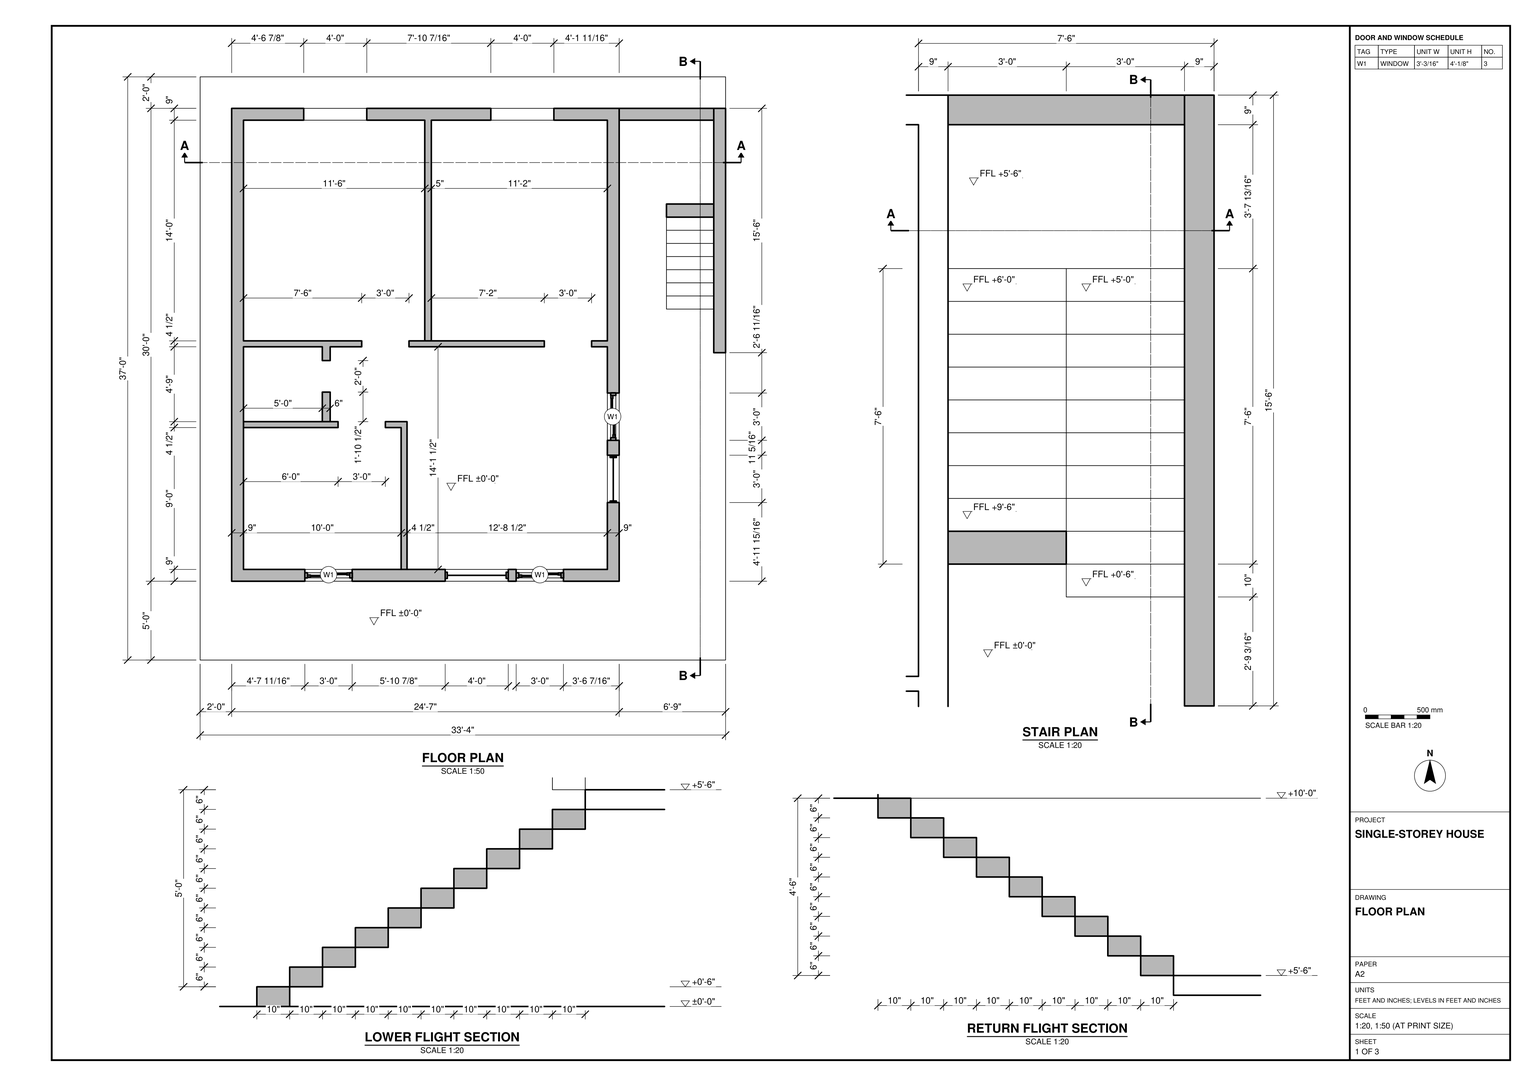
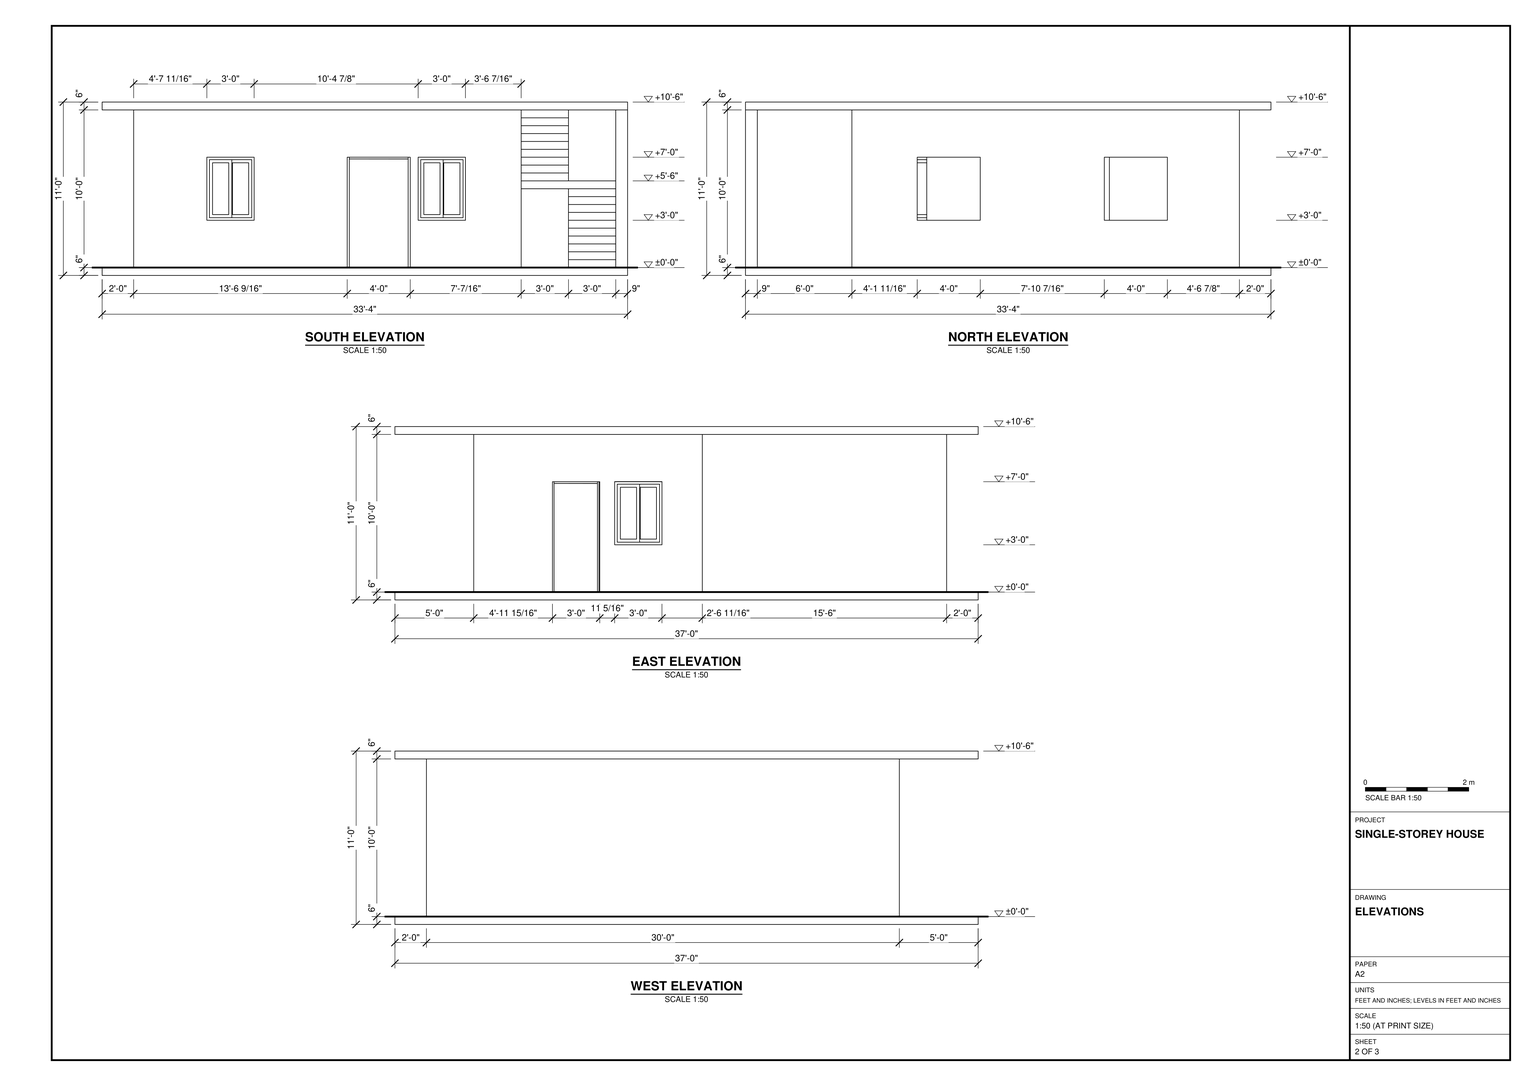
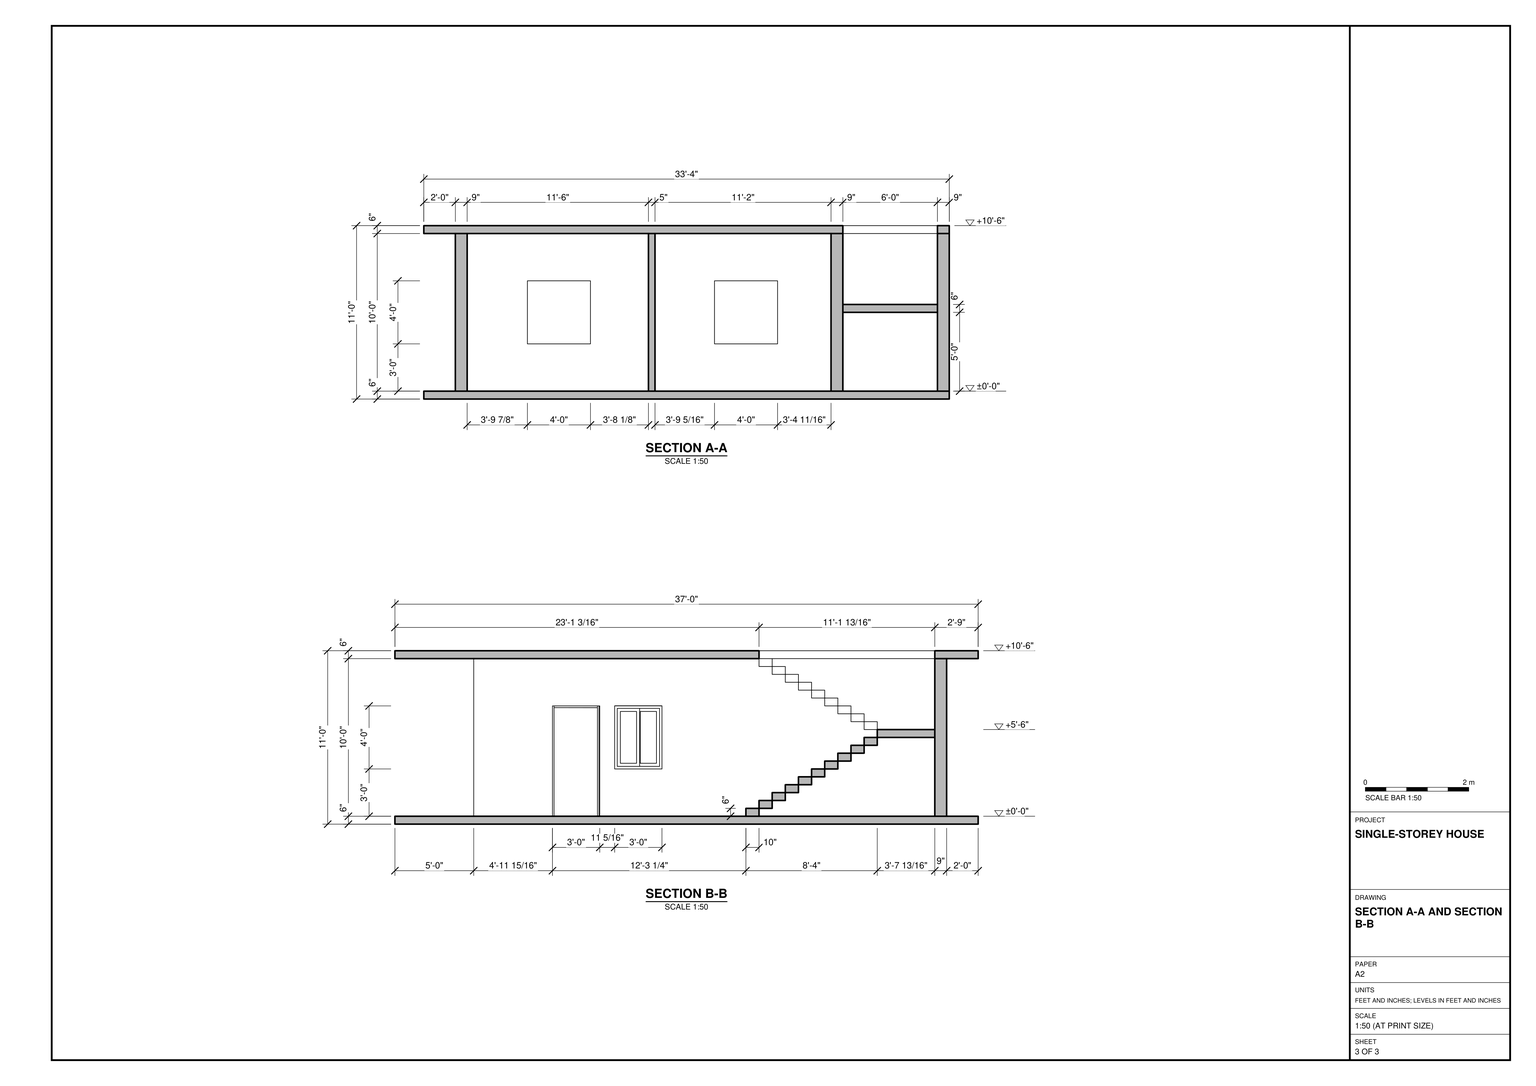
Build the single-storey house in SketchUp from task_files/diagram_01.pdf. Work in feet and inches. The overall dimensions, including the projecting slabs, are 33'-4" east to west, 37'-0" north to south and 11'-0" high. Use ±0'-0" as the finished ground-floor level.

Set out the 24'-7" by 30'-0" enclosed house on the floor slab. Follow the plan for the two rooms across the north end, the smaller subdivided spaces on the west and the larger space at the southeast. Use 9" exterior walls and follow the individual partition thicknesses, including the 5" divider between the north rooms. Cut the passage openings through the partitions. Place the south entrance between two sliding windows, with another doorway and sliding window on the east wall. Reproduce the two plain openings on the north elevation and leave the west wall uninterrupted.

Model the floor slab and flat roof slab, including their projections beyond the walls. At the northeast, build the stair between the house and the outer stair wall. Use the stair plan and sections to connect the parallel flights at the +5'-6" landing and form the roof opening for the return flight.

Keep walls, slabs, roof, stair and any individual furniture or joinery pieces in separate groups or components. Use components for repeated parts. Any decor or loose items may be suitable library components. Save one SketchUp model as output_files/single_storey_house_with_an_external_return_stair.skp.

# SketchUp Ruby script. Lengths in inches.
U = 1.inch
M = Sketchup.active_model
def pt(a) = Geom::Point3d.new(a.map { |v| v * U })
def face(e, loops, mat)
  f = e.add_face(loops[0].map { |a| pt(a) })
  loops[1..].each { |l| e.add_face(l.map { |a| pt(a) }).erase! }
  f.material = f.back_material = mat if mat
  f
end
# faces: each face lists its corners as indices into pts; further lists are holes
def faces(e, pts, list, mat = nil) = list.each { |f| face(e, (f[0].is_a?(Array) ? f : [f]).map { |l| l.map { |i| pts[i] } }, mat) }
# xy, xz, yz: faces in a plane at the given z, y or x. An outline is a flat list of corners, or four numbers for a rectangle; further outlines are holes
def ring(l) = l.size == 4 ? [[l[0], l[1]], [l[2], l[1]], [l[2], l[3]], [l[0], l[3]]] : l.each_slice(2).to_a
def flat(e, list, mat, &to3) = list.each { |f| face(e, (f[0].is_a?(Array) ? f : [f]).map { |l| ring(l).map { |u, v| to3.(u, v) } }, mat) }
def xy(e, z, list, mat = nil) = flat(e, list, mat) { |x, y| [x, y, z] }
def xz(e, y, list, mat = nil) = flat(e, list, mat) { |x, z| [x, y, z] }
def yz(e, x, list, mat = nil) = flat(e, list, mat) { |y, z| [x, y, z] }
def lines(e, pts, list) = list.each { |a, b| e.add_line(pt(pts[a]), pt(pts[b])) }
# prism: a flat outline (further loops are holes) pulled along v
def prism(e, loops, v, mat = nil)
  f = face(e, loops, mat); d = Geom::Vector3d.new(v.map { |x| x * U })
  f.pushpull(f.normal.samedirection?(d) ? d.length : -d.length)
end
def box(e, o, s, mat = nil) = prism(e, [[o, [o[0] + s[0], o[1], o[2]], [o[0] + s[0], o[1] + s[1], o[2]], [o[0], o[1] + s[1], o[2]]]], [0, 0, s[2]], mat)
def at(x, y, z, deg = 0) = Geom::Transformation.translation(pt([x, y, z])) * Geom::Transformation.rotation(ORIGIN, Z_AXIS, deg.degrees)
def axes(o, x, y, z) = Geom::Transformation.new([*x, 0, *y, 0, *z, 0, *pt(o).to_a, 1])
def part(name) = M.definitions.add(name)
# library, detail: a bought-in or finely detailed component or shape, given as its bounding box
def library(name, o, s) = part(name).tap { |d| box(d.entities, o, s) }
def detail(e, o, s) = box(e.add_group.entities, o, s)
def put(e, d, t, mat = nil) = e.add_instance(d, t).tap { |i| i.material = mat if mat }
def group(e, t, mat = nil) = e.add_group.tap { |g| g.transformation = t; g.material = mat if mat }.entities
root = M.entities
M.materials.add("Polis06_194").color = [79, 50, 36]
c1 = library("Sliding Window",[0,0,0],[36.16,4.93,48.1])
c2 = library("Sliding Window\#1",[0,0,0],[36.16,4.93,48.1])
c3 = part("Flush door")
xy(c3.entities,0,[[0,0,4.72,1.18],[0,34.25,4.72,35.43]],"Polis06_194")
xy(c3.entities,85.26,[[0,1.18,4.72,34.25]],"Polis06_194")
xy(c3.entities,86.61,[[0,0,4.72,35.43]],"Polis06_194")
xz(c3.entities,0,[[0,0,4.72,86.61]],"Polis06_194")
xz(c3.entities,1.18,[[0,0,2.36,85.26],[2.36,0,4.72,85.26]],"Polis06_194")
xz(c3.entities,34.25,[[0,0,4.72,85.26]],"Polis06_194")
xz(c3.entities,35.43,[[0,0,4.72,86.61]],"Polis06_194")
yz(c3.entities,0,[[0,0,1.18,86.61],[34.25,0,35.43,86.61],[1.18,85.26,34.25,86.61]],"Polis06_194")
yz(c3.entities,2.36,[[1.18,0,34.25,0,34.25,85.21,1.18,85.26]],"Polis06_194")
yz(c3.entities,4.72,[[0,0,1.18,86.61],[34.25,0,35.43,86.61],[1.18,85.26,34.25,86.61]],"Polis06_194")
c4 = part("Flush door \#1")
xy(c4.entities,0,[[0,0,4.72,1.18],[0,34.25,4.72,35.43]],"Polis06_194")
xy(c4.entities,85.26,[[0,1.18,4.72,34.25]],"Polis06_194")
xy(c4.entities,86.61,[[0,0,4.72,35.43]],"Polis06_194")
xz(c4.entities,0,[[0,0,4.72,86.61]],"Polis06_194")
xz(c4.entities,1.18,[[0,0,2.36,85.26],[2.36,0,4.72,85.26]],"Polis06_194")
xz(c4.entities,34.25,[[0,0,4.72,85.26]],"Polis06_194")
xz(c4.entities,35.43,[[0,0,4.72,86.61]],"Polis06_194")
yz(c4.entities,0,[[0,0,1.18,86.61],[34.25,0,35.43,86.61],[1.18,85.26,34.25,86.61]],"Polis06_194")
yz(c4.entities,2.36,[[1.18,0,34.25,0,34.25,85.21,1.18,85.26]],"Polis06_194")
yz(c4.entities,4.72,[[0,0,1.18,86.61],[34.25,0,35.43,86.61],[1.18,85.26,34.25,86.61]],"Polis06_194")
c5 = part("Group\#2")
box(c5.entities,[0,0,0],[36,10,6])
xy(root,0,[[391,234,400,420],[319,411,391,420]])
xy(root,120,[[391,234,400,420],[319,411,391,420]])
xz(root,234,[[391,0,400,120]])
xz(root,411,[[319,0,391,120]])
xz(root,420,[[319,0,391,120],[391,0,400,120]])
yz(root,319,[[411,0,420,120]])
yz(root,391,[[234,0,411,120],[411,0,420,120]])
yz(root,400,[[234,0,420,120]])
put(root,c1,at(240.5625,62.53,36))
put(root,c1,at(79.72,62.53,36))
put(root,c2,at(316.47,167.28,36,90))
put(root,c3,axes([312.14,119.94,0],[1,0,0],[0,1,0],[0,0,0.96982]))
put(root,c4,axes([186.5625,66.86,0],[0,-1,0],[1.35467,0,0],[0,0,0.96982]))
g1 = group(root,at(355,367.1875,60))
box(g1,[-36,0,0],[72,43.8125,6])
put(root,c5,axes([319,277.1875,120],[1,0,0],[0,1,0],[0,0,-1]))
put(root,c5,axes([319,317.1875,96],[1,0,0],[0,1,0],[0,0,-1]))
put(root,c5,axes([319,357.1875,72],[1,0,0],[0,1,0],[0,0,-1]))
put(root,c5,axes([319,337.1875,84],[1,0,0],[0,1,0],[0,0,-1]))
put(root,c5,axes([319,307.1875,102],[1,0,0],[0,1,0],[0,0,-1]))
put(root,c5,axes([319,327.1875,90],[1,0,0],[0,1,0],[0,0,-1]))
put(root,c5,axes([319,297.1875,108],[1,0,0],[0,1,0],[0,0,-1]))
put(root,c5,axes([319,287.1875,114],[1,0,0],[0,1,0],[0,0,-1]))
put(root,c5,axes([319,347.1875,78],[1,0,0],[0,1,0],[0,0,-1]))
put(root,c5,at(355,277.1875,6))
put(root,c5,at(355,317.1875,30))
put(root,c5,at(355,357.1875,54))
put(root,c5,at(355,337.1875,42))
put(root,c5,at(355,307.1875,24))
put(root,c5,at(355,327.1875,36))
put(root,c5,at(355,297.1875,18))
put(root,c5,at(355,287.1875,12))
put(root,c5,at(355,347.1875,48))
put(root,c5,at(355,267.1875,0))
g2 = group(root,at(24,60,0))
xy(g2,0,[[0,0,0,360,295,360,295,95.94,286,95.94,286,178.5,274,178.5,274,183,286,183,286,351,152,351,152,183,147,183,147,351,9,351,9,183,99,183,99,178.5,75,178.5,75,168,69,168,69,178.5,9,178.5,9,9,162.5625,9,162.5625,0],[210.5625,0,210.5625,9,286,9,286,59.94,295,59.94,295,0],[129,9,129,117,117,117,117,121.5,133.5,121.5,133.5,9],[9,117,81,121.5],[69,121.5,75,144],
  [135,178.5,238,183]])
xy(g2,36,[[55.72,0,91.72,9],[216.5625,0,252.5625,9],[286,107.28,295,143.28],[54.85,351,102.85,360],[197.29,351,245.29,360]])
xy(g2,84,[[55.72,0,91.72,9],[162.5625,0,210.5625,9],[216.5625,0,252.5625,9],[286,59.94,295,95.94],[286,107.28,295,143.28],
  [81,117,117,121.5],[69,144,75,168],[99,178.5,135,183],[238,178.5,274,183],[54.85,351,102.85,360],
  [197.29,351,245.29,360]])
xy(g2,120,[[[0,0,295,360],[9,183,9,351,147,351,147,183,152,183,152,351,286,351,286,183],[9,9,9,117,129,117,129,9,133.5,9,133.5,121.5,9,121.5,9,178.5,69,178.5,69,121.5,75,121.5,75,178.5,286,178.5,286,9]]])
xz(g2,0,[[[0,0,162.5625,0,162.5625,84,210.5625,84,210.5625,0,295,0,295,120,0,120],[55.72,36,91.72,84],[216.5625,36,252.5625,84]]])
xz(g2,9,[[[9,0,129,120],[55.72,36,91.72,84]],[129,0,133.5,120],[[133.5,0,133.5,120,286,120,286,0,210.5625,0,210.5625,84,162.5625,84,162.5625,0],[216.5625,36,252.5625,84]]])
xz(g2,59.94,[[286,0,295,84]])
xz(g2,95.94,[[286,0,295,84]])
xz(g2,107.28,[[286,36,295,84]])
xz(g2,117,[[9,0,81,0,81,84,117,84,117,0,129,0,129,120,9,120]])
xz(g2,121.5,[[9,0,69,120],[69,0,75,120],[75,0,75,120,133.5,120,133.5,0,117,0,117,84,81,84,81,0]])
xz(g2,143.28,[[286,36,295,84]])
xz(g2,144,[[69,0,75,84]])
xz(g2,168,[[69,0,75,84]])
xz(g2,178.5,[[9,0,69,120],[75,0,99,0,99,84,135,84,135,0,238,0,238,84,274,84,274,0,286,0,286,120,75,120]])
xz(g2,183,[[9,0,9,120,147,120,147,0,135,0,135,84,99,84,99,0],[147,0,152,120],[152,0,152,120,286,120,286,0,274,0,274,84,238,84,238,0]])
xz(g2,351,[[[9,0,147,120],[54.85,36,102.85,84]],[[152,0,286,120],[197.29,36,245.29,84]]])
xz(g2,360,[[[0,0,295,120],[54.85,36,102.85,84],[197.29,36,245.29,84]]])
yz(g2,0,[[0,0,360,120]])
yz(g2,9,[[9,0,117,120],[117,0,121.5,84],[121.5,0,178.5,120],[183,0,351,120]])
yz(g2,54.85,[[351,36,360,84]])
yz(g2,55.72,[[0,36,9,84]])
yz(g2,69,[[121.5,0,121.5,120,178.5,120,178.5,0,168,0,168,84,144,84,144,0]])
yz(g2,75,[[121.5,0,144,0,144,84,168,84,168,0,178.5,0,178.5,120,121.5,120]])
yz(g2,81,[[117,0,121.5,84]])
yz(g2,91.72,[[0,36,9,84]])
yz(g2,99,[[178.5,0,183,84]])
yz(g2,102.85,[[351,36,360,84]])
yz(g2,117,[[117,0,121.5,84]])
yz(g2,129,[[9,0,117,120]])
yz(g2,133.5,[[9,0,121.5,120]])
yz(g2,135,[[178.5,0,183,84]])
yz(g2,147,[[183,0,351,120]])
yz(g2,152,[[183,0,351,120]])
yz(g2,162.5625,[[0,0,9,84]])
yz(g2,197.29,[[351,36,360,84]])
yz(g2,210.5625,[[0,0,9,84]])
yz(g2,216.5625,[[0,36,9,84]])
yz(g2,238,[[178.5,0,183,84]])
yz(g2,245.29,[[351,36,360,84]])
yz(g2,252.5625,[[0,36,9,84]])
yz(g2,274,[[178.5,0,183,84]])
yz(g2,286,[[[9,0,59.94,0,59.94,84,95.94,84,95.94,0,178.5,0,178.5,120,9,120],[107.28,36,143.28,84]],[183,0,351,120]])
yz(g2,295,[[[0,0,59.94,0,59.94,84,95.94,84,95.94,0,360,0,360,120,0,120],[107.28,36,143.28,84]]])
p = [[295,95.94,0],[295,59.94,0],[286,59.94,0],[286,95.94,0],[162.5625,9,0],[210.5625,9,0],
  [162.5625,0,0],[210.5625,0,0]]
lines(g2,p,[[0,1],[2,3],[4,5],[6,7]])
g3 = group(root,at(0,0,-6))
box(g3,[0,0,0],[400,444,6])
g4 = group(root,at(0,0,120))
prism(g4,[[[400,0,0],[0,0,0],[0,444,0],[400,444,0]],[[319,411,0],[319,277.1875,0],[391,277.1875,0],[391,411,0]]],[0,0,6])
